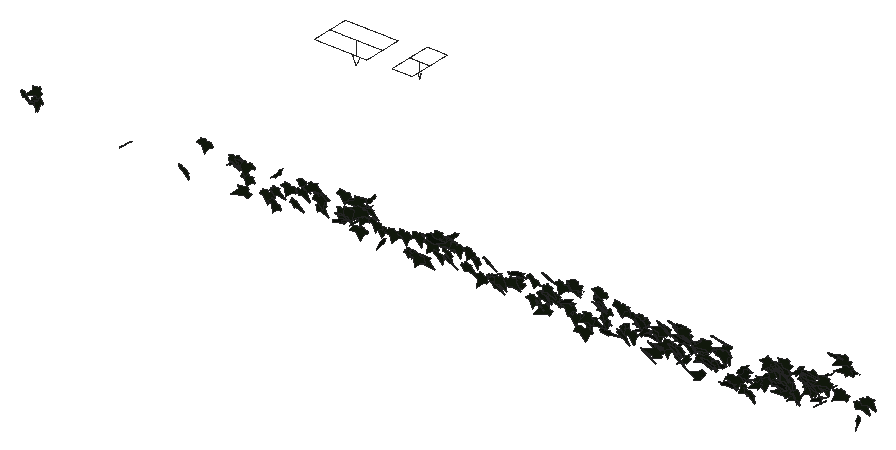
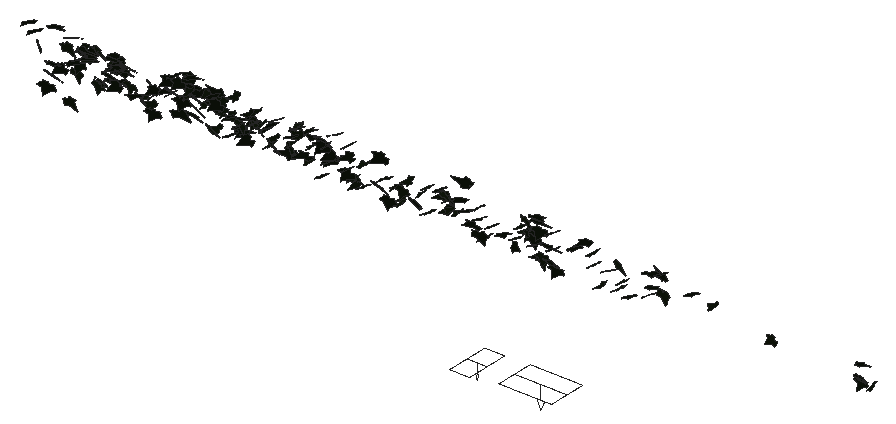
# SketchUp Ruby script. Lengths in millimetres.
U = 1.mm
M = Sketchup.active_model
def pt(a) = Geom::Point3d.new(a.map { |v| v * U })
def face(e, loops, mat)
  f = e.add_face(loops[0].map { |a| pt(a) })
  loops[1..].each { |l| e.add_face(l.map { |a| pt(a) }).erase! }
  f.material = f.back_material = mat if mat
  f
end
# faces: each face lists its corners as indices into pts; further lists are holes
def faces(e, pts, list, mat = nil) = list.each { |f| face(e, (f[0].is_a?(Array) ? f : [f]).map { |l| l.map { |i| pts[i] } }, mat) }
# xy, xz, yz: faces in a plane at the given z, y or x. An outline is a flat list of corners, or four numbers for a rectangle; further outlines are holes
def ring(l) = l.size == 4 ? [[l[0], l[1]], [l[2], l[1]], [l[2], l[3]], [l[0], l[3]]] : l.each_slice(2).to_a
def flat(e, list, mat, &to3) = list.each { |f| face(e, (f[0].is_a?(Array) ? f : [f]).map { |l| ring(l).map { |u, v| to3.(u, v) } }, mat) }
def xy(e, z, list, mat = nil) = flat(e, list, mat) { |x, y| [x, y, z] }
def xz(e, y, list, mat = nil) = flat(e, list, mat) { |x, z| [x, y, z] }
def yz(e, x, list, mat = nil) = flat(e, list, mat) { |y, z| [x, y, z] }
def lines(e, pts, list) = list.each { |a, b| e.add_line(pt(pts[a]), pt(pts[b])) }
# prism: a flat outline (further loops are holes) pulled along v
def prism(e, loops, v, mat = nil)
  f = face(e, loops, mat); d = Geom::Vector3d.new(v.map { |x| x * U })
  f.pushpull(f.normal.samedirection?(d) ? d.length : -d.length)
end
def box(e, o, s, mat = nil) = prism(e, [[o, [o[0] + s[0], o[1], o[2]], [o[0] + s[0], o[1] + s[1], o[2]], [o[0], o[1] + s[1], o[2]]]], [0, 0, s[2]], mat)
def at(x, y, z, deg = 0) = Geom::Transformation.translation(pt([x, y, z])) * Geom::Transformation.rotation(ORIGIN, Z_AXIS, deg.degrees)
def axes(o, x, y, z) = Geom::Transformation.new([*x, 0, *y, 0, *z, 0, *pt(o).to_a, 1])
def part(name) = M.definitions.add(name)
# library, detail: a bought-in or finely detailed component or shape, given as its bounding box
def library(name, o, s) = part(name).tap { |d| box(d.entities, o, s) }
def detail(e, o, s) = box(e.add_group.entities, o, s)
def put(e, d, t, mat = nil) = e.add_instance(d, t).tap { |i| i.material = mat if mat }
def group(e, t, mat = nil) = e.add_group.tap { |g| g.transformation = t; g.material = mat if mat }.entities
root = M.entities
M.materials.add("efeu1").color = [18, 25, 13]
c1 = part("ivyleaf_9")
p = [[39.1,54.8,31.7],[34.5,51.8,30.2],[-5.3,25.2,17.3],[-17.9,28.3,20.9],[-21.6,21.7,17],[-20.2,4.3,5.3],
  [-22.9,-0.3,2.5],[-17.1,-4,-0.6],[-2,-2.1,-1.2],[-0.7,-15.4,-10.1],[16.6,-22.3,-16.7],[21.1,-15.1,-12.5],
  [32.7,-10.7,-11],[46.1,-1.8,-6.6],[30.8,11.2,3.8]]
faces(c1.entities,p,[[0,1,2,3,4,5,6,7,8,9,10,11,12,13,14]],"efeu1")
c2 = part("Group259\#1")
p = [[0,0,0],[0,0,-168.3],[-48,0,-168.3],[312.5,-232.4,0],[-312.5,-232.4,0],[312.5,232.4,0],
  [312.5,0,0],[-312.5,232.4,0],[48,0,-168.3],[-312.5,0,0],[0,0,-272.5]]
lines(c2.entities,p,[[0,1],[1,2],[3,4],[5,6],[7,5],[1,8],[9,0],[0,6],[8,10],[4,9],[6,3],[2,10],
  [9,7]])
c3 = part("Rectangle Light\#5")
put(c3.entities,c2,at(0,0,0))
c4 = part("Group261\#1")
p = [[0,0,0],[0,0,-117.5],[-18.3,0,-117.5],[119,-261.3,0],[-119,-261.3,0],[119,261.3,0],
  [119,0,0],[-119,261.3,0],[18.3,0,-117.5],[-119,0,0],[0,0,-190.1]]
lines(c4.entities,p,[[0,1],[1,2],[3,4],[5,6],[7,5],[1,8],[9,0],[0,6],[8,10],[4,9],[6,3],[2,10],
  [9,7]])
c5 = part("Rectangle Light\#6")
put(c5.entities,c4,at(0,0,0))
put(root,c1,axes([4927.4,509,5461.8],[1.36686,-0.99518,-0.77753],[-0.31153,0.81357,-1.1925],[2.3833,0.6771,0.29005]))
put(root,c1,axes([6872.9,568.1,5438.7],[-0.65461,-1.37252,0.18283],[-0.10287,-0.17494,-1.41493],[2.63324,-0.34803,-0.00983]))
put(root,c1,axes([5020.7,524.2,5460.2],[1.58605,0.45387,-1.07421],[-1.72688,-0.57701,-0.94772],[-1.39419,1.23104,-0.04816]))
put(root,c1,axes([8821.7,585.9,5439.5],[1.96548,0.91922,0.01181],[-0.18149,0.12479,-1.37366],[-1.74016,1.02522,0.15661]))
put(root,c1,axes([6613.4,471.8,5449.5],[-2.53132,-0.32152,0.3936],[-0.55707,-0.41686,-1.3296],[0.79074,-1.32293,0.32331]))
put(root,c1,axes([6493.9,483.2,5464.6],[2.32111,-0.70142,-0.48697],[-0.75869,0.28316,-1.40621],[1.43716,1.28232,0.04415]))
put(root,c1,axes([4042.5,579.7,5447.3],[1.78774,1.02694,0.18715],[0.19788,0.15848,-1.39142],[-1.97678,0.94459,0.02998]))
put(root,c1,axes([9046.5,407.8,5457],[0.64167,-1.36506,0.4324],[0.33856,-0.40085,-1.40417],[2.70409,0.37411,0.0732]))
put(root,c1,axes([3515,567.4,5468],[1.63154,-1.00618,-0.51554],[-0.26246,0.54909,-1.30099],[2.13563,0.83617,0.23396]))
put(root,c1,axes([3217.9,575.5,5448.6],[-0.87334,-1.3419,0.0499],[0.01056,-0.05463,-1.41801],[2.55565,-0.45834,0.02291]))
put(root,c1,axes([8228.5,535.9,5466],[-2.10008,0.73053,-0.46601],[0.49107,-0.4433,-1.30589],[-1.57433,-1.11276,0.2143]))
put(root,c1,axes([8138.8,494.2,5455.5],[1.03328,-1.16136,0.64439],[0.5833,-0.56781,-1.28157],[2.45953,0.62256,0.03322]))
put(root,c1,axes([3415,442.1,5459.4],[-0.79226,-1.1614,0.84505],[-0.14683,-0.86048,-1.22061],[2.72963,-0.38338,0.17962]))
put(root,c1,axes([4630.3,512.9,5466.2],[-0.79605,0.49888,-1.28167],[1.32578,-1.07824,-0.64703],[-2.25697,-0.80934,0.07198]))
put(root,c1,axes([5937.2,534.6,5467],[1.30604,-1.23226,-0.32982],[-0.14913,0.33309,-1.40751],[2.42321,0.68465,0.09114]))
put(root,c1,axes([4320.5,547.1,5470.1],[-1.10858,-1.25982,-0.26242],[0.5823,0.14421,-1.37146],[2.37893,-0.62238,0.21341]))
put(root,c1,axes([7302.1,448.7,5464.5],[1.95423,-0.1813,1.04982],[1.99307,-0.09613,-1.04087],[0.37254,1.46534,0.06161]))
put(root,c1,axes([9005.7,419,5457.9],[-0.92624,-0.5933,1.17746],[-0.8086,-1.11759,-0.73875],[2.3755,-0.61176,0.20764]))
put(root,c1,axes([6411.6,531.3,5470.8],[-0.87931,-1.30272,0.30419],[-0.13659,-0.29722,-1.38187],[2.54236,-0.46653,0.03097]))
put(root,c1,axes([471.6,522.1,5479.6],[1.22143,1.09817,0.29768],[-0.07309,0.44685,-1.44695],[-1.38619,0.94408,0.3386]))
put(root,c1,axes([498.2,537.3,5497.4],[-1.05679,-0.79984,-0.90298],[1.12455,0.2782,-1.13067],[0.94931,-1.21997,0.33418]))
put(root,c1,axes([5132.2,455.9,5481.9],[-0.25581,-0.56577,-1.35578],[2.26173,0.75854,-0.43436],[1.6438,-1.13174,0.38665]))
put(root,c1,axes([1625.3,408.9,5466.5],[1.11558,0.65304,1.08802],[0.91244,0.99569,-0.85591],[-2.23607,0.7321,0.19356]))
put(root,c1,axes([7073.2,484.9,5481.2],[0.16787,-1.21713,0.73176],[0.45994,-0.70961,-1.20942],[2.66343,0.19925,0.16273]))
put(root,c1,axes([8867.7,573.6,5482.1],[0.88287,-1.1148,0.75016],[1.12188,-0.54433,-1.17343],[2.2981,0.694,0.28465]))
put(root,c1,axes([9503.3,568.7,5487.1],[0.54687,1.26951,0.59267],[-0.03824,0.60868,-1.29406],[-2.66618,0.25166,0.14013]))
put(root,c1,axes([5831.3,493.7,5507.2],[-2.51105,0.17367,-0.70505],[1.33272,-0.08253,-1.33074],[-0.36561,-1.49367,-0.00845]))
put(root,c1,axes([9475.1,567.3,5475.6],[1.19031,-0.46193,-1.19881],[1.83615,-0.71158,0.77752],[-1.61462,-1.14976,0.00043]))
put(root,c1,axes([7977.2,423.8,5476.4],[-1.36525,0.11468,1.30667],[-2.49049,-0.16508,-0.70391],[0.17183,-1.48146,0.17958]))
put(root,c1,axes([6044.9,581.5,5488.9],[1.32979,1.22453,-0.12666],[-0.10744,-0.11362,-1.40983],[-2.3405,0.70095,-0.00725]))
put(root,c1,axes([7959.4,557.5,5490.1],[-0.60185,-1.40158,0.10554],[0.01389,-0.10981,-1.43647],[2.675,-0.31477,0.0312]))
put(root,c1,axes([4242.9,582.1,5491.1],[-0.23428,1.38655,0.24644],[-0.03499,0.24578,-1.392],[-2.68,-0.12442,-0.00337]))
put(root,c1,axes([523.7,523.4,5515.9],[-1.4153,-0.43014,-0.81683],[0.94844,0.25228,-1.23694],[0.60739,-1.39619,0.02814]))
put(root,c1,axes([3288.7,572.8,5516.7],[1.41312,-1.04326,-0.62084],[-0.11002,0.69654,-1.2396],[2.30789,0.67199,0.32104]))
put(root,c1,axes([5566.6,559,5515.8],[1.24003,-1.18582,-0.46502],[0.25423,0.58306,-1.29966],[2.41081,0.54846,0.37624]))
put(root,c1,axes([3104.9,394.1,5502.9],[-2.18096,-0.38162,0.74556],[-1.25127,-0.37291,-1.2014],[0.98755,-1.31529,0.1243]))
put(root,c1,axes([9084.8,523,5503.7],[-2.21144,0.81927,-0.14576],[0.25237,-0.06485,-1.42155],[-1.56348,-1.16927,-0.02328]))
put(root,c1,axes([318.8,561.2,5505],[1.08796,-1.17666,-0.0689],[-0.00047,0.08611,-1.4755],[1.43798,0.89027,0.05164]))
put(root,c1,axes([9502.8,1020.6,5529.3],[-0.52032,1.23285,-0.73202],[-0.03488,-0.74815,-1.25318],[-2.72858,-0.22553,0.15561]))
put(root,c1,axes([5143.4,403.8,5517.2],[-1.16908,-1.2618,0.47841],[-0.20737,-0.47755,-1.39944],[2.55989,-0.61494,0.10512]))
put(root,c1,axes([7862.5,454.3,5523.5],[2.69408,-0.23149,-0.35118],[-0.64962,0.08821,-1.43402],[0.46775,1.4558,0.03105]))
put(root,c1,axes([8576.3,557.7,5524.7],[0.08998,0.67777,-1.2711],[-1.67082,-0.99476,-0.56307],[-2.17362,0.79271,0.38021]))
put(root,c1,axes([9087.7,575.7,5529.1],[-1.22291,-1.13933,-0.53327],[0.54515,0.45057,-1.30777],[2.33125,-0.70303,0.02608]))
put(root,c1,axes([2390.4,344,5520.2],[0.49454,-1.28174,0.64002],[0.42579,-0.60618,-1.3048],[2.69317,0.3312,0.08876]))
put(root,c1,axes([4215.4,577.3,5520.2],[0.98897,1.27378,0.34985],[0.02733,0.37048,-1.37021],[-2.51389,0.50513,0.12274]))
put(root,c1,axes([9518.4,552.4,5523.7],[-2.60951,0.32287,-0.19373],[0.3312,-0.10538,-1.40725],[-0.63549,-1.38072,0.0621]))
put(root,c1,axes([9782.2,548,5521],[0.0052,1.42249,0.21712],[-0.14541,0.21696,-1.42047],[-2.73478,-0.00883,0.07594]))
put(root,c1,axes([5905.9,524.8,5531],[1.06353,-1.30448,-0.29792],[-0.07188,0.30735,-1.41662],[2.54559,0.55368,0.08447]))
put(root,c1,axes([4146.2,588.3,5479],[-2.54454,0.42942,-0.05658],[-0.09872,0.02352,1.40424],[0.81841,1.33797,-0.00652]))
put(root,c1,axes([7481.1,513.4,5546.2],[1.33309,-1.11799,-0.5801],[-0.33987,0.56892,-1.31206],[2.37293,0.70956,0.13797]))
put(root,c1,axes([6478.2,536,5543.7],[1.38696,-1.13378,-0.45794],[-0.29655,0.44265,-1.34389],[2.30821,0.73814,0.10251]))
put(root,c1,axes([7330.2,437.3,5526.8],[0.00922,0.97409,1.11854],[-0.03063,1.11851,-0.974],[-2.82273,-0.00895,0.01422]))
put(root,c1,axes([2989.5,573.9,5535.2],[-0.92094,-1.23962,0.49954],[-0.03468,-0.5251,-1.32071],[2.54337,-0.45602,0.16287]))
put(root,c1,axes([7714.2,567.7,5530.2],[2.68428,0.09144,0.13178],[0.24895,0.01925,-1.41332],[-0.17668,1.41641,0.0107]))
put(root,c1,axes([7115.7,457.1,5522.8],[0.15043,-0.13601,-1.43122],[1.3927,1.23761,-0.07719],[2.35521,-0.72315,0.13706]))
put(root,c1,axes([9429.2,519.4,5534.1],[-2.12119,0.05815,0.86777],[-1.65428,-0.12262,-1.10817],[0.0565,-1.40719,0.13243]))
put(root,c1,axes([7519.1,423.8,5543.3],[1.14315,-1.35241,0.32448],[0.2681,-0.29247,-1.47976],[2.63334,0.61687,0.0098]))
put(root,c1,axes([8903.9,387.9,5564.8],[-1.68537,-1.00647,-0.67325],[0.95272,0.45518,-1.33891],[2.09842,-1.01502,0.06716]))
put(root,c1,axes([7520.7,513,5547.2],[-1.84197,1.04536,-0.08556],[0.1185,-0.05896,-1.42459],[-1.99267,-0.96981,-0.00562]))
put(root,c1,axes([8440.5,551.9,5550.7],[-2.70619,0.17774,0.05329],[-0.10582,-0.01523,-1.43281],[-0.33692,-1.42283,0.022]))
put(root,c1,axes([7249.7,212.4,5577.9],[-1.53201,-1.02477,-0.70081],[1.12193,0.41957,-1.29062],[2.07944,-0.98136,0.18002]))
put(root,c1,axes([6848.3,503.3,5561.7],[-0.76832,-1.34636,0.39865],[-0.13159,-0.39523,-1.40485],[2.66912,-0.40704,0.04549]))
put(root,c1,axes([5299.7,497.5,5564.7],[0.0458,-1.2772,0.64928],[0.37965,-0.64006,-1.26646],[2.70027,0.11165,0.16705]))
put(root,c1,axes([6805.4,496.8,5581.7],[-0.35974,-1.24217,-0.72214],[0.48091,0.68827,-1.25005],[2.69195,-0.28896,0.12681]))
put(root,c1,axes([5399.2,486.9,5565.5],[2.01516,-1.02786,-0.12884],[-0.11325,0.12358,-1.47492],[1.96827,1.05946,0.04704]))
put(root,c1,axes([6049,461.4,5583.2],[0.32551,-1.33042,-0.62015],[-0.14431,0.61551,-1.34136],[2.78989,0.18707,0.00297]))
put(root,c1,axes([7933.1,244.2,5570.9],[1.85238,-1.07747,0.38027],[0.45393,-0.29694,-1.45183],[2.1267,1.00187,-0.02133]))
put(root,c1,axes([10313.3,460.2,5587.1],[-1.40932,0.50176,-1.1883],[1.93198,-0.61869,-0.89382],[-1.51463,-1.25604,-0.03443]))
put(root,c1,axes([4580.6,547.4,5569.6],[-0.70889,-1.29911,0.39715],[0.2388,-0.44295,-1.33124],[2.57437,-0.31664,0.23285]))
put(root,c1,axes([6244.8,545.2,5568.6],[-2.59105,0.48171,-0.02484],[0.02891,-0.03153,-1.44392],[-0.91755,-1.36128,0.02465]))
put(root,c1,axes([9255.9,587.6,5569.7],[1.49046,0.78513,0.86915],[1.08698,0.65683,-1.10794],[-1.94616,0.96814,0.04682]))
put(root,c1,axes([5960.7,479,5574.9],[1.05049,1.22692,0.44872],[0.1312,0.45909,-1.34008],[-2.48288,0.54336,0.11904]))
put(root,c1,axes([7300.9,476.5,5580.1],[-0.19084,-1.29004,0.74225],[0.06732,-0.74578,-1.29141],[2.83179,-0.06921,0.08072]))
put(root,c1,axes([6550.3,540.7,5573.2],[2.51,0.59296,-0.04033],[-0.07266,-0.01344,-1.44599],[-1.12879,1.31938,0.00339]))
put(root,c1,axes([4730.9,559.4,5570.4],[-1.29472,-1.24426,0.0029],[-0.02517,0.00392,-1.41803],[2.36796,-0.68028,-0.01348]))
put(root,c1,axes([9288.8,543.2,5591.5],[-0.33904,-1.23294,-0.6519],[0.22431,0.64154,-1.24555],[2.64486,-0.21246,0.02207]))
put(root,c1,axes([7125.1,382.5,5582.8],[0.52113,-1.40281,0.24989],[0.03816,-0.25065,-1.42901],[2.71159,0.27313,-0.02792]))
put(root,c1,axes([8911.1,222.4,5586.5],[2.66336,0.44335,0.25844],[0.47701,0.06456,-1.46789],[-0.85226,1.42161,-0.01393]))
put(root,c1,axes([5355.1,550.8,5591.1],[0.31603,-1.25244,0.68003],[0.3983,-0.65578,-1.25887],[2.68293,0.24489,0.10679]))
put(root,c1,axes([7645.4,416.4,5592.4],[-0.12687,-1.45743,-0.11975],[-0.02811,0.12054,-1.45882],[2.78299,-0.06522,-0.02019]))
put(root,c1,axes([9771.2,514.7,5590.5],[1.24008,1.27703,0.1716],[0.17214,0.14649,-1.43358],[-2.44624,0.65768,-0.01389]))
put(root,c1,axes([6175.6,453.5,5617],[0.68245,-1.16255,-0.85228],[0.1635,0.89393,-1.18322],[2.73858,0.23634,0.28303]))
put(root,c1,axes([8079.7,435.9,5596.2],[-2.00985,0.85098,0.45147],[-1.09226,-0.01773,-1.30902],[-1.47251,-1.14836,0.35477]))
put(root,c1,axes([8594.8,449.7,5598.7],[-0.14456,-1.30748,0.69233],[0.43014,-0.69536,-1.2884],[2.78267,0.03956,0.23513]))
put(root,c1,axes([4349.3,577.9,5594.4],[-1.27633,-1.19066,0.37379],[0.01378,-0.42805,-1.3505],[2.37506,-0.63736,0.20871]))
put(root,c1,axes([9149.7,538.8,5595.2],[0.69777,1.20329,0.62989],[-0.21707,0.67741,-1.22767],[-2.57576,0.26888,0.2741]))
put(root,c1,axes([8619.8,230.5,5546.6],[0.12577,0.00927,1.487],[-2.47862,-0.71808,0.06235],[1.36602,-1.3038,-0.02377]))
put(root,c1,axes([6583.6,524.9,5598.5],[-0.08746,-1.44786,-0.0496],[-0.10144,0.05128,-1.44755],[2.75531,-0.04407,-0.05487]))
put(root,c3,at(2426.6,2861.3,5793.7))
put(root,c1,axes([4251.4,527.2,5608.1],[-2.31722,0.26805,0.70615],[-1.37671,-0.02834,-1.23646],[-0.41366,-1.40721,0.15941]))
put(root,c1,axes([8122.7,427,5604.6],[1.27543,-1.24736,0.22064],[0.2159,-0.18952,-1.41595],[2.40115,0.67961,0.01012]))
put(root,c1,axes([4133.8,536.2,5616.5],[0.18566,-1.36693,-0.36073],[0.25279,0.36885,-1.36178],[2.67871,0.05993,0.15352]))
put(root,c1,axes([9430.8,547.1,5613.5],[-2.65697,-0.08857,-0.26621],[0.50962,-0.01731,-1.39846],[0.15938,-1.42111,0.03362]))
put(root,c1,axes([3488.7,557.4,5613],[-1.25526,-1.19456,0.45534],[0.00794,-0.51437,-1.3434],[2.43304,-0.61462,0.2393]))
put(root,c1,axes([4860.9,548.6,5607.7],[-0.38293,-1.43414,0.09331],[-0.00336,-0.09397,-1.44814],[2.73523,-0.2009,0.01128]))
put(root,c1,axes([9708,1055.5,5625],[2.27478,0.80782,-0.26787],[-0.49017,-0.09685,-1.44125],[-1.54382,1.22105,0.0629]))
put(root,c1,axes([559.1,492.2,5623.9],[-1.49714,-0.12721,0.85092],[-0.97937,-0.36399,-1.21213],[0.37765,-1.44827,0.2299]))
put(root,c1,axes([7865.6,544.8,5618.6],[-0.11544,-1.44042,0.20084],[-0.03455,-0.20025,-1.44166],[2.76771,-0.06258,-0.00962]))
put(root,c1,axes([9018.5,432.3,5619.4],[-2.0635,0.91326,-0.10998],[0.21257,-0.03803,-1.41695],[-1.73771,-1.08913,-0.04274]))
put(root,c1,axes([6821.6,436.6,5622.2],[1.87625,0.73634,0.76259],[1.13738,0.47409,-1.23033],[-1.66637,1.15268,0.01888]))
put(root,c1,axes([3625.9,550.5,5632.4],[0.80753,-1.3398,-0.3065],[0.14213,0.34277,-1.39498],[2.61191,0.39557,0.17067]))
put(root,c1,axes([5222.1,520.5,5628.5],[-1.50935,-1.07983,0.55135],[-0.39507,-0.52817,-1.33301],[2.27346,-0.80868,0.1344]))
put(root,c1,axes([8910.7,476.7,5615.1],[-0.0027,0.02126,-1.50798],[-0.62395,1.47191,0.02106],[2.80163,0.32783,0.00324]))
put(root,c1,axes([3969.8,407,5650.6],[0.83856,-1.25473,-0.59867],[-0.32924,0.57366,-1.32962],[2.62533,0.47272,0.02448]))
put(root,c1,axes([2801.3,576.3,5630.8],[0.12756,1.41664,-0.05834],[-0.00155,-0.05837,-1.41823],[-2.69844,0.067,-0.00194]))
put(root,c1,axes([8208.2,404.1,5640.7],[0.16905,-1.27822,0.71794],[0.75297,-0.67167,-1.24479],[2.68666,0.26867,0.30369]))
put(root,c1,axes([5707.6,540,5638.8],[0.0711,-1.28682,0.66912],[-0.02591,-0.66962,-1.28703],[2.76025,0.02686,-0.02932]))
put(root,c1,axes([7860.7,526.2,5641.7],[-0.11363,1.38799,0.42023],[-0.2125,0.41494,-1.38637],[-2.75184,-0.08935,0.08971]))
put(root,c1,axes([6716,429.9,5651.4],[0.45014,-1.35729,-0.41351],[0.09055,0.42657,-1.37294],[2.6989,0.21207,0.11503]))
put(root,c1,axes([4583,470.8,5656.1],[-0.70498,-1.23949,0.69554],[0.19787,-0.74047,-1.2642],[2.69778,-0.26959,0.27448]))
put(root,c1,axes([8389.5,560,5649.1],[-2.16947,0.87237,0.01427],[0.02676,0.04184,-1.43481],[-1.66031,-1.13923,-0.04177]))
put(root,c1,axes([7750.9,428.1,5659.9],[1.23959,1.2331,0.39354],[0.3709,0.34211,-1.39449],[-2.43538,0.67974,-0.01207]))
put(root,c1,axes([8509.5,553.5,5662.8],[1.95723,0.989,-0.20213],[-0.32325,-0.1149,-1.42636],[-1.89377,1.04175,0.03457]))
put(root,c1,axes([9748.9,645.8,5676.9],[-0.48457,-1.25388,-0.64372],[0.2881,0.62603,-1.27929],[2.66698,-0.29545,0.02124]))
put(root,c1,axes([7259.9,299.9,5659.2],[-1.26302,-0.73428,1.15007],[-1.31961,-0.91998,-0.98747],[2.23661,-0.95744,0.06683]))
put(root,c1,axes([7784.9,416.6,5652.5],[0.02586,0.2771,-1.43012],[-1.18153,1.2949,0.245],[2.50805,0.60716,0.13016]))
put(root,c1,axes([4353.1,561.4,5671.5],[0.64069,1.3601,-0.31395],[-0.08545,-0.31223,-1.4008],[-2.65523,0.33823,-0.03067]))
put(root,c1,axes([4361.4,532.3,5684.5],[1.4257,-0.92857,-0.8013],[-0.66307,0.73916,-1.18227],[2.23814,0.81049,0.16017]))
put(root,c1,axes([8193.5,442,5628.6],[0.8678,1.31362,0.59506],[-0.83096,-0.46906,1.37002],[2.61582,-0.5848,0.2378]))
put(root,c1,axes([9392.8,535.8,5671.4],[0.01047,-1.40369,-0.17962],[0.25231,0.17934,-1.39746],[2.68144,-0.01139,0.1322]))
put(root,c1,axes([9731.8,510,5669.5],[-1.49992,-0.63932,1.06645],[-0.90125,-1.01314,-0.95731],[2.1881,-0.85555,0.33673]))
put(root,c1,axes([8577,335.5,5694.5],[-0.84756,-0.97085,-0.99995],[1.14615,0.81266,-1.05721],[2.39213,-0.73336,0.15225]))
put(root,c1,axes([7964.7,531.4,5652.2],[-1.03857,0.23019,1.33071],[-2.57014,-0.10494,-0.53563],[0.02137,-1.43442,0.25274]))
put(root,c1,axes([8269.9,517.7,5677.4],[0.65254,-1.26926,0.60559],[0.51016,-0.55292,-1.31063],[2.62746,0.42258,0.10408]))
put(root,c1,axes([7295.7,488.5,5676.7],[-1.0606,-1.37609,0.09712],[-0.01237,-0.10213,-1.4843],[2.62546,-0.55638,0.03224]))
put(root,c1,axes([3914.9,495.3,5688.1],[-0.52426,-1.3882,-0.32804],[0.08463,0.32559,-1.41513],[2.71346,-0.27836,-0.01924]))
put(root,c1,axes([7702.4,503.7,5677.5],[-1.1834,1.2979,0.10009],[-0.08696,0.08909,-1.43916],[-2.47597,-0.62347,0.00271]))
put(root,c1,axes([6421.8,510.6,5683.5],[-0.54325,-1.11664,0.90899],[0.25261,-0.94314,-1.11691],[2.72864,-0.135,0.28437]))
put(root,c1,axes([8665.2,539,5678.2],[0.15681,-1.44543,0.00768],[-0.00023,-0.0077,-1.44778],[2.75098,0.08239,-0.00056]))
put(root,c1,axes([7931.3,532.6,5695.3],[2.29769,-0.795,-0.27537],[-0.32235,0.24211,-1.44155],[1.56846,1.21438,0.10713]))
put(root,c1,axes([8445.8,492.4,5688.8],[-2.72145,0.25709,-0.07317],[0.07911,-0.17951,-1.44299],[-0.50253,-1.42051,0.16911]))
put(root,c5,at(3143.4,2908.6,5793.7))
put(root,c1,axes([9795.5,965.4,5694.9],[-2.29225,0.71168,0.47101],[-0.91332,0.10892,-1.39169],[-1.34313,-1.28865,0.1425]))
put(root,c1,axes([9738.9,500.7,5710.5],[-2.15816,-0.57806,-0.70492],[1.33125,0.1698,-1.26445],[1.11268,-1.32437,0.14557]))
put(root,c1,axes([9258.9,550.3,5698.3],[-2.24195,-0.77493,-0.29532],[0.52928,0.11417,-1.4089],[1.48692,-1.20906,0.05624]))
put(root,c1,axes([5342.5,520,5712],[0.55395,-1.201,-0.72711],[0.34869,0.76872,-1.19638],[2.64917,0.14995,0.30951]))
put(root,c1,axes([5072.1,476,5696.5],[0.06927,-1.47553,-0.11222],[-0.06809,0.11134,-1.47561],[2.81551,0.03899,-0.03293]))
put(root,c1,axes([7214.8,465.8,5688.5],[0.27978,-0.85265,1.23638],[1.32462,-1.06217,-0.81526],[2.53293,0.64965,0.28978]))
put(root,c1,axes([8351.6,398.1,5696.8],[-0.23097,-1.0892,1.01192],[0.57373,-1.01222,-1.05337],[2.77075,0.1188,0.30247]))
put(root,c1,axes([4410.6,558.2,5715.7],[-0.76526,1.00373,-0.95074],[0.436,-0.92808,-1.07669],[-2.59486,-0.45195,0.09948]))
put(root,c1,axes([7691,551,5696.7],[-0.22663,-1.3992,0.28998],[-0.06794,-0.28798,-1.40421],[2.71869,-0.12383,-0.01092]))
put(root,c1,axes([9435.9,354.7,5701.3],[2.56839,0.48708,-0.11313],[-0.19954,-0.04275,-1.43472],[-0.93054,1.35357,-0.0046]))
put(root,c1,axes([3915.8,455.7,5702.2],[0.06642,-1.49386,0.11893],[0.03484,-0.11853,-1.49419],[2.8519,0.03624,0.01548]))
put(root,c1,axes([7606.5,521.9,5704.8],[0.57154,-1.40547,0.3462],[0.13389,-0.33898,-1.43719],[2.75158,0.30843,-0.00198]))
put(root,c1,axes([8690.3,548.2,5710.3],[-2.04661,0.89327,0.40312],[-0.97667,-0.00338,-1.36142],[-1.58902,-1.14842,0.31757]))
put(root,c1,axes([5668.7,516.3,5708.7],[-1.05223,-1.07256,0.79441],[-0.15531,-0.8311,-1.17888],[2.53548,-0.49602,0.25747]))
put(root,c1,axes([5865.5,493.7,5706.4],[1.70513,-1.1274,0.1164],[0.09149,-0.11044,-1.43971],[2.15513,0.89668,-0.03097]))
put(root,c1,axes([9622.7,575.4,5718.4],[-1.79099,-1.04549,-0.26852],[0.52199,0.11295,-1.40097],[1.98693,-0.97206,0.12601]))
put(root,c1,axes([4416.8,547.7,5717.1],[1.38132,-1.2362,-0.16537],[0.23415,0.26136,-1.41381],[2.36212,0.697,0.23685]))
put(root,c1,axes([9589.6,542.5,5728.4],[2.29963,-0.61085,-0.49034],[-0.31118,0.68487,-1.2561],[1.45796,1.10967,0.50532]))
put(root,c1,axes([9302.5,538.9,5718.4],[1.91064,-0.97791,0.29204],[0.33064,-0.23992,-1.4006],[1.91403,1.01762,-0.04957]))
put(root,c1,axes([8660.4,252.8,5720.1],[2.78569,-0.23984,-0.10882],[-0.20274,0.02287,-1.4832],[0.45843,1.46755,0.00533]))
put(root,c1,axes([3026.5,486.4,5728.8],[-1.45835,-1.26593,-0.27277],[0.25203,0.23868,-1.47974],[2.45169,-0.77756,-0.01014]))
put(root,c1,axes([7491.5,494,5746.1],[0.98941,-0.7931,-1.17638],[-0.22954,1.22363,-0.87826],[2.69042,0.39606,0.35769]))
put(root,c1,axes([9360.2,569.6,5719.9],[-0.00931,-1.42792,-0.03492],[-0.09846,0.03507,-1.42698],[2.71664,-0.00362,-0.05184]))
put(root,c1,axes([3378.5,543.9,5731.6],[-1.48345,1.18919,-0.29571],[0.33078,-0.23963,-1.4218],[-2.30861,-0.79847,-0.0137]))
put(root,c1,axes([10311.7,487.2,5746.5],[0.29661,-1.25597,-0.75891],[0.25712,0.77222,-1.25025],[2.78098,0.06256,0.19654]))
put(root,c1,axes([9239.6,558.4,5727.9],[1.58434,-1.1673,-0.14836],[0.09404,0.21625,-1.42421],[2.2375,0.81746,0.16491]))
put(root,c1,axes([9244.7,558.3,5721.2],[0.049,-1.44015,0.00221],[-0.00026,-0.00222,-1.44038],[2.74089,0.02575,-0.00017]))
put(root,c1,axes([8485.4,500.4,5728.1],[0.09904,-1.12236,0.94769],[0.41923,-0.9316,-1.1154],[2.76408,0.18151,0.13522]))
put(root,c1,axes([9257.9,553.7,5746.2],[0.02152,-0.87813,-1.1424],[1.01269,1.06423,-0.81278],[2.54849,-0.41548,0.33262]))
put(root,c1,axes([5236.1,518.5,5746.8],[0.43125,-0.81784,-1.18014],[0.3536,1.2014,-0.7969],[2.70969,-0.02662,0.29181]))
put(root,c1,axes([8224.8,518.5,5729.1],[-2.34145,-0.69047,0.30807],[-0.46275,-0.19581,-1.40988],[1.36253,-1.25305,0.05056]))
put(root,c1,axes([9919.8,538,5748.2],[-0.69757,1.25461,-0.65412],[-0.03726,-0.68014,-1.29355],[-2.69256,-0.31562,0.18736]))
put(root,c1,axes([5527.2,482,5734.2],[-0.18296,-1.44563,-0.17645],[0.04753,0.17517,-1.44876],[2.77134,-0.09844,0.0132]))
put(root,c1,axes([5395.9,547.8,5732],[2.42485,-0.60733,0.25545],[0.49837,-0.04354,-1.40959],[1.15065,1.29872,0.0722]))
put(root,c1,axes([2480.9,573,5728.6],[-1.05099,-1.3096,0.07111],[-0.03792,-0.06877,-1.42124],[2.49581,-0.55252,0.00835]))
put(root,c1,axes([6677.6,372.5,5754.4],[0.95166,-1.35154,-0.44614],[-0.03607,0.46651,-1.43449],[2.70853,0.48109,0.13765]))
put(root,c1,axes([3643,528.9,5744.4],[1.18881,-1.28792,-0.23648],[-0.03197,0.2541,-1.42828],[2.49194,0.61768,0.09449]))
put(root,c1,axes([9737.1,465,5737.8],[2.04619,-1.05416,-0.02386],[-0.03295,0.01642,-1.50571],[2.00652,1.07527,-0.0004]))
put(root,c1,axes([7748.1,430.6,5741.1],[-0.12107,-1.23456,0.76645],[0.08999,-0.76853,-1.234],[2.76413,-0.02906,0.07375]))
put(root,c1,axes([2895.2,463.4,5699.3],[-0.36659,0.41185,1.41968],[1.19832,-1.27246,0.45457],[2.54537,0.65837,-0.00954]))
put(root,c1,axes([6858.5,526,5743.9],[2.65994,0.45178,-0.09469],[-0.17455,-0.02413,-1.46881],[-0.861,1.40061,0.00524]))
put(root,c1,axes([2898.9,481.8,5753.3],[-0.18952,-1.46951,-0.22114],[0.24726,0.21218,-1.46846],[2.81744,-0.11747,0.114]))
put(root,c1,axes([6835.6,523.9,5761.6],[1.34018,-1.21921,-0.41464],[-0.02803,0.46492,-1.39208],[2.45075,0.67203,0.21082]))
put(root,c1,axes([9238.7,531,5715.9],[-2.56044,0.39426,-0.44857],[-0.82139,0.12231,1.40191],[0.7856,1.41286,0.00381]))
put(root,c1,axes([8119.5,487.5,5757.7],[2.37917,-0.73499,-0.26237],[-0.38732,0.17129,-1.44949],[1.43389,1.26579,0.0438]))
put(root,c1,axes([6526.5,543.3,5748.8],[2.42658,-0.65604,0.19068],[0.33,-0.07978,-1.43386],[1.25768,1.28671,0.00832]))
put(root,c1,axes([6280.1,376.2,5762.2],[2.48852,0.58379,0.43393],[0.73041,0.20459,-1.43166],[-1.17602,1.3624,0.02905]))
put(root,c1,axes([5421.2,562.8,5758.3],[-1.14244,1.30334,0.11699],[-0.57899,-0.01381,-1.40712],[-2.42226,-0.61141,0.28116]))
put(root,c1,axes([9316.5,557,5774.3],[0.14868,-1.30015,-0.61932],[-0.05753,0.61862,-1.30248],[2.74024,0.08353,0.00626]))
put(root,c1,axes([9202.3,543.6,5772.6],[-2.59788,-0.32845,-0.38418],[0.91173,-0.48787,-1.28499],[0.30678,-1.33147,0.56561]))
put(root,c1,axes([8232.4,384.6,5734.1],[0.23341,-0.45475,1.37077],[1.98479,-0.92383,-0.39978],[1.90153,1.0201,0.24903]))
put(root,c1,axes([8094.5,550.7,5762.5],[2.70015,0.26826,0.01661],[0.03039,0.00496,-1.44388],[-0.51063,1.41883,0.0019]))
put(root,c1,axes([4267.9,546.9,5766.8],[1.57574,1.16374,0.19694],[0.20011,0.16689,-1.42817],[-2.23739,0.83452,0.01097]))
put(root,c1,axes([8750.1,397,5774.1],[-0.22133,-1.4569,-0.19574],[-0.03673,0.19784,-1.46112],[2.79744,-0.11267,-0.03467]))
put(root,c1,axes([8213.3,484.5,5790.3],[0.18485,-1.25033,-0.79343],[-0.15848,0.78927,-1.25396],[2.81385,0.12659,-0.0185]))
put(root,c1,axes([3797,462.4,5778.7],[0.33714,-0.46759,-1.38586],[0.13462,1.39709,-0.46234],[2.7804,-0.01095,0.19043]))
put(root,c1,axes([8048.1,522.9,5780.9],[1.8166,-1.06604,0.38231],[0.77081,-0.14562,-1.4172],[2.01288,1.01785,0.19767]))
put(root,c1,axes([7234.3,460.3,5776.9],[-0.25318,-1.10095,0.95258],[0.24005,-0.96166,-1.09384],[2.76035,-0.01735,0.1825]))
put(root,c1,axes([4153.4,549.9,5780.7],[-0.79693,-1.34091,0.34966],[0.0297,-0.36981,-1.39951],[2.63719,-0.40104,0.12142]))
put(root,c1,axes([7236.3,435.4,5790.7],[1.36574,-1.20347,-0.40129],[-0.26319,0.38408,-1.39917],[2.40003,0.72696,0.07492]))
put(root,c1,axes([4475.1,392.3,5780.2],[-2.30928,-0.79616,0.1212],[-0.19441,-0.06525,-1.45125],[1.52032,-1.21766,-0.00148]))
put(root,c1,axes([7467.9,486.7,5789.8],[-0.55608,-1.40869,0.33526],[0.24796,-0.36621,-1.42516],[2.74472,-0.25232,0.19667]))
put(root,c1,axes([9569.5,563,5776.9],[1.52465,-0.44513,1.10199],[1.84295,-0.52605,-0.91644],[1.31145,1.25674,0.00672]))
put(root,c1,axes([10387.3,482,5812.4],[0.31686,-1.2202,-0.82634],[0.29794,0.84154,-1.2111],[2.78884,0.04873,0.22327]))
put(root,c1,axes([4403.7,485.9,5792.2],[-2.30396,0.18215,0.78668],[-1.52807,-0.12042,-1.20764],[-0.16381,-1.4387,0.20068]))
put(root,c1,axes([9695.8,562.7,5769.4],[-0.86892,0.23798,1.34108],[-2.21995,0.66199,-0.51457],[-1.33844,-1.25248,-0.01715]))
put(root,c1,axes([6923.4,522.4,5795.9],[-2.80436,-0.05512,-0.05772],[0.11667,-0.09832,-1.4711],[0.09726,-1.47135,0.10047]))
put(root,c1,axes([9381.6,548,5745.6],[0.04766,-1.45181,-0.02128],[-0.02873,-0.02154,1.45194],[-2.76323,-0.02482,-0.01546]))
put(root,c1,axes([9769.3,961.2,5799.8],[-2.67143,-0.19848,0.24245],[-0.44463,-0.07865,-1.41692],[0.39739,-1.42226,0.04452]))
put(root,c1,axes([9389.8,560.3,5802.3],[-2.56083,-0.20134,0.42441],[-0.76608,-0.16956,-1.3566],[0.46084,-1.40066,0.10322]))
put(root,c1,axes([8578.1,514.8,5813.4],[2.6764,0.06522,-0.35296],[-0.68312,0.25859,-1.38228],[0.00146,1.42664,0.26669]))
put(root,c1,axes([7203.3,540.2,5810],[-1.33413,-1.1796,0.63665],[-0.35155,-0.62659,-1.36434],[2.52678,-0.71,0.14633]))
put(root,c1,axes([8602.3,383.9,5801],[-1.8753,-0.3661,1.03841],[-1.75522,-0.48682,-1.04675],[1.14473,-1.34618,0.09614]))
put(root,c1,axes([9605.5,963.6,5798.6],[2.7193,-0.04326,0.00196],[0.00383,0.00172,-1.42946],[0.08232,1.42881,0.00178]))
put(root,c1,axes([9907.1,509.9,5814.9],[-2.29876,-0.45087,0.75555],[-0.81564,-0.81923,-1.17397],[1.46246,-1.16559,0.53287]))
put(root,c1,axes([10164.5,426.3,5813],[-2.28324,-0.73423,0.4595],[-0.71471,-0.26645,-1.40622],[1.48547,-1.25674,0.02969]))
put(root,c1,axes([6852.8,409.9,5815.1],[-1.27791,-1.20045,0.4815],[-0.11516,-0.51277,-1.36278],[2.45893,-0.64789,0.18641]))
put(root,c1,axes([7997,404.5,5813.9],[1.77643,-1.1679,0.18815],[0.24037,-0.13991,-1.49502],[2.23853,0.94183,0.01122]))
put(root,c1,axes([9580.9,508.7,5817.8],[-1.53915,1.1905,-0.05372],[0.06076,-0.04325,-1.43921],[-2.26726,-0.80935,-0.0021]))
put(root,c1,axes([4468.2,547.1,5823.4],[-0.87769,1.34459,0.30251],[-0.09906,0.30178,-1.42068],[-2.62111,-0.46165,-0.0476]))
put(root,c1,axes([5304,345.1,5800.4],[0.98706,-0.22234,1.37144],[2.35017,-0.59711,-0.56379],[1.21182,1.33913,-0.02368]))
